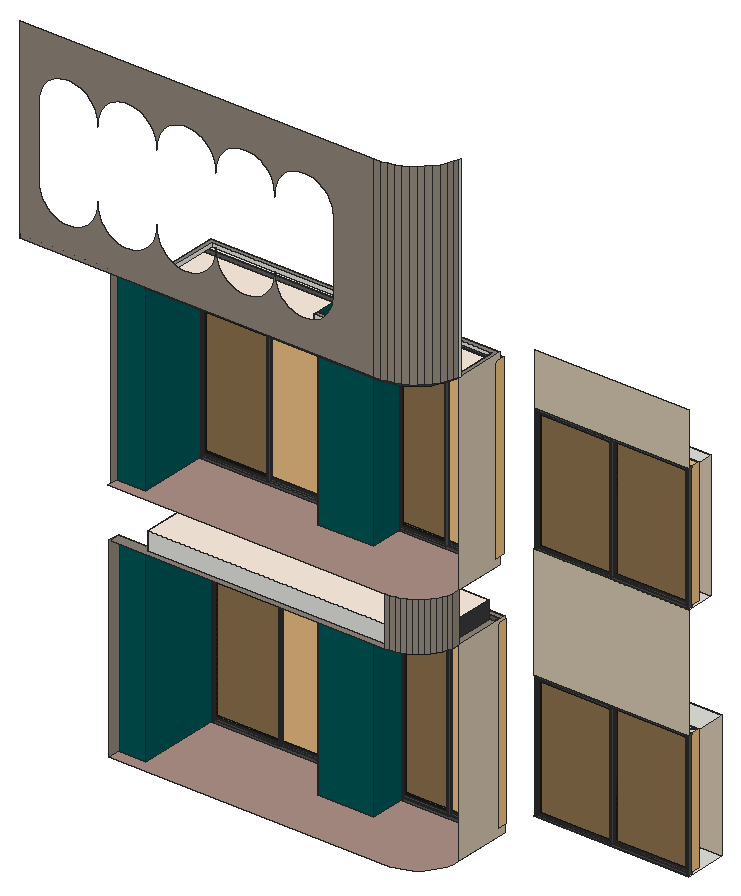
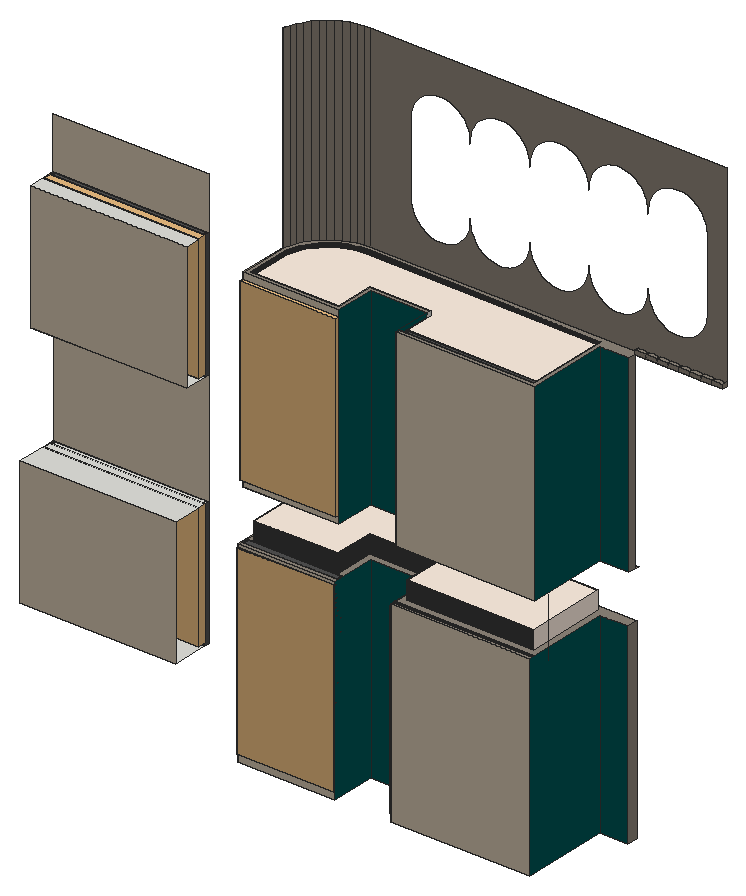
# SketchUp Ruby script. Lengths in inches.
U = 1.inch
M = Sketchup.active_model
def pt(a) = Geom::Point3d.new(a.map { |v| v * U })
def face(e, loops, mat)
  f = e.add_face(loops[0].map { |a| pt(a) })
  loops[1..].each { |l| e.add_face(l.map { |a| pt(a) }).erase! }
  f.material = f.back_material = mat if mat
  f
end
# faces: each face lists its corners as indices into pts; further lists are holes
def faces(e, pts, list, mat = nil) = list.each { |f| face(e, (f[0].is_a?(Array) ? f : [f]).map { |l| l.map { |i| pts[i] } }, mat) }
# xy, xz, yz: faces in a plane at the given z, y or x. An outline is a flat list of corners, or four numbers for a rectangle; further outlines are holes
def ring(l) = l.size == 4 ? [[l[0], l[1]], [l[2], l[1]], [l[2], l[3]], [l[0], l[3]]] : l.each_slice(2).to_a
def flat(e, list, mat, &to3) = list.each { |f| face(e, (f[0].is_a?(Array) ? f : [f]).map { |l| ring(l).map { |u, v| to3.(u, v) } }, mat) }
def xy(e, z, list, mat = nil) = flat(e, list, mat) { |x, y| [x, y, z] }
def xz(e, y, list, mat = nil) = flat(e, list, mat) { |x, z| [x, y, z] }
def yz(e, x, list, mat = nil) = flat(e, list, mat) { |y, z| [x, y, z] }
def lines(e, pts, list) = list.each { |a, b| e.add_line(pt(pts[a]), pt(pts[b])) }
# prism: a flat outline (further loops are holes) pulled along v
def prism(e, loops, v, mat = nil)
  f = face(e, loops, mat); d = Geom::Vector3d.new(v.map { |x| x * U })
  f.pushpull(f.normal.samedirection?(d) ? d.length : -d.length)
end
def box(e, o, s, mat = nil) = prism(e, [[o, [o[0] + s[0], o[1], o[2]], [o[0] + s[0], o[1] + s[1], o[2]], [o[0], o[1] + s[1], o[2]]]], [0, 0, s[2]], mat)
def at(x, y, z, deg = 0) = Geom::Transformation.translation(pt([x, y, z])) * Geom::Transformation.rotation(ORIGIN, Z_AXIS, deg.degrees)
def axes(o, x, y, z) = Geom::Transformation.new([*x, 0, *y, 0, *z, 0, *pt(o).to_a, 1])
def part(name) = M.definitions.add(name)
# library, detail: a bought-in or finely detailed component or shape, given as its bounding box
def library(name, o, s) = part(name).tap { |d| box(d.entities, o, s) }
def detail(e, o, s) = box(e.add_group.entities, o, s)
def put(e, d, t, mat = nil) = e.add_instance(d, t).tap { |i| i.material = mat if mat }
def group(e, t, mat = nil) = e.add_group.tap { |g| g.transformation = t; g.material = mat if mat }.entities
root = M.entities
M.materials.add("Brown Tiles 240cm").color = [174, 145, 135]
M.materials.add("Glass_Tinted_Gray").color = [0, 0, 0]
M.materials["Glass_Tinted_Gray"].alpha = 0.125
M.materials.add("Heather_Band").color = [142, 133, 122]
M.materials.add("Lily_Blonde").color = [209, 194, 173]
M.materials.add("[0135_DarkGray]").color = [81, 81, 81]
M.materials.add("[Color C02]").color = [255, 240, 226]
M.materials.add("[Color H08]").color = [0, 84, 84]
M.materials.add("[Color M07]").color = [58, 58, 58]
M.materials.add("[Mirror 02]").color = [229, 229, 229]
M.materials.add("[Terrazzo Light Blue]").color = [196, 214, 227]
c1 = library("Window curtains",[0,0,0],[14.46,147.43,135.83])
c2 = part("PENTEK_RP Fineline 50S_Sliding_DoorCase_E1")
box(c2.entities,[0,0,0],[1.51,3.66,99.27],"[0135_DarkGray]")
c3 = part("PENTEK_RP Fineline 50S_SlidingDooe_Case_E2")
box(c3.entities,[0,0,0],[96.25,3.66,1.51],"[0135_DarkGray]")
c4 = part("pentek_RP Fineline 50S_SlidingDoor_Case")
put(c4.entities,c2,at(97.76,0,0))
put(c4.entities,c3,at(1.51,0,0))
put(c4.entities,c2,at(0,0,0))
put(c4.entities,c3,at(1.51,0,97.76))
c5 = part("PENTEK_RP Fineline 50S_SlidingDoor_GlazingBead_2")
box(c5.entities,[0,0,0],[0.56,0.59,94.39],"[0135_DarkGray]")
c6 = part("PENTEK_RP Fineline 50S_SlidingDoor_Glass")
box(c6.entities,[0,0,0],[46.58,0.16,94.39],"Glass_Tinted_Gray")
c7 = part("PENTEK_RP Fineline 50S_SlidingDoor_GlazingBead")
box(c7.entities,[0,0,0],[45.47,0.59,0.56],"[0135_DarkGray]")
c8 = part("PENTEK_RP Fineline 50S_SlidingDoor_Leaf_E1")
xy(c8.entities,0,[[0,0,0.93,1.97],[0.93,1.57,1.49,1.97]],"[0135_DarkGray]")
xy(c8.entities,96.25,[[0,0,0.93,0,0.93,1.57,1.49,1.57,1.49,1.97,0,1.97]],"[0135_DarkGray]")
xz(c8.entities,0,[[0,0,0.93,96.25]],"[0135_DarkGray]")
xz(c8.entities,1.57,[[0.93,0,1.49,95.32],[0.93,95.32,1.49,96.25]],"[0135_DarkGray]")
xz(c8.entities,1.97,[[0,0,1.49,96.25]],"[0135_DarkGray]")
yz(c8.entities,0,[[0,0,1.97,96.25]],"[0135_DarkGray]")
yz(c8.entities,0.93,[[0,0,1.57,0.93],[0,0.93,1.57,95.32],[0,95.32,1.57,96.25]],"[0135_DarkGray]")
yz(c8.entities,1.49,[[1.57,0,1.97,95.32],[1.57,95.32,1.97,96.25]],"[0135_DarkGray]")
c9 = part("PENTEK_RP Fineline 50S_SlidingDoor_Leaf_E2")
xy(c9.entities,0,[[0,0,0,1.57,0.56,1.57,0.56,1.97,46.02,1.97,46.02,1.57,46.58,1.57,46.58,0]],"[0135_DarkGray]")
xy(c9.entities,0.93,[[0,0,46.58,1.57]],"[0135_DarkGray]")
xy(c9.entities,1.49,[[0.56,1.57,46.02,1.97]],"[0135_DarkGray]")
xz(c9.entities,0,[[0,0,46.58,0.93]],"[0135_DarkGray]")
xz(c9.entities,1.57,[[0,0,0.56,0.93],[46.02,0,46.58,0.93],[0.56,0.93,46.02,1.49]],"[0135_DarkGray]")
xz(c9.entities,1.97,[[0.56,0,46.02,1.49]],"[0135_DarkGray]")
yz(c9.entities,0,[[0,0,1.57,0.93]],"[0135_DarkGray]")
yz(c9.entities,0.56,[[1.57,0,1.97,0.93],[1.57,0.93,1.97,1.49]],"[0135_DarkGray]")
yz(c9.entities,46.02,[[1.57,0,1.97,0.93],[1.57,0.93,1.97,1.49]],"[0135_DarkGray]")
yz(c9.entities,46.58,[[0,0,1.57,0.93]],"[0135_DarkGray]")
c10 = part("PENTEK_RP Fineline S_SlidingDoor_Leaf1")
put(c10.entities,c5,at(0.93,0,0.93))
put(c10.entities,c5,at(46.96,0,0.93))
put(c10.entities,c6,at(1.49,1.42,0.93))
put(c10.entities,c7,at(1.49,0,0.93))
put(c10.entities,c6,at(1.49,0.59,0.93),"[Terrazzo Light Blue]")
put(c10.entities,c8,at(0,0,0))
put(c10.entities,c8,axes([48.44,0,0],[-1,0,0],[0,1,0],[0,0,1]))
put(c10.entities,c9,axes([0.93,0,96.25],[1,0,0],[0,1,0],[0,0,-1]))
put(c10.entities,c9,at(0.93,0,0))
put(c10.entities,c7,at(1.49,0,94.77))
c11 = part("PENTEK_RP Fineline 50S_SlidingDoor_Leaf2")
put(c11.entities,c6,at(1.49,1.42,0.93))
put(c11.entities,c7,at(1.49,0,94.77))
put(c11.entities,c5,at(46.96,0,0.93))
put(c11.entities,c6,at(1.49,0.59,0.93),"[Mirror 02]")
put(c11.entities,c5,at(0.93,0,0.93))
put(c11.entities,c8,at(0,0,0))
put(c11.entities,c8,axes([48.44,0,0],[-1,0,0],[0,1,0],[0,0,1]))
put(c11.entities,c7,at(1.49,0,0.93))
put(c11.entities,c9,axes([0.93,0,96.25],[1,0,0],[0,1,0],[0,0,-1]))
put(c11.entities,c9,at(0.93,0,0))
c12 = part("PENTEK - Slimmest Steel Sliding Door / Window\#1")
put(c12.entities,c4,at(0,-1.88,-0.09))
put(c12.entities,c10,at(1.51,-2.27,1.42))
put(c12.entities,c11,at(49.32,-0.3,1.42))
c13 = part("Group\#18")
put(c13.entities,c1,axes([0,8.14,5.43],[0,-0.42,0],[1.40442,0,0],[0,0,0.9702]))
put(c13.entities,c12,axes([0,2.27,0.13],[2.0736,0,0],[0,1,0],[0,0,1.4]))
c14 = library("White+Curtain+Sketchup",[0,-2.58,0],[59,4.99,76.02])
c15 = part("Group\#8")
put(c15.entities,c12,axes([0.12,3.91,0.18],[2.38,0,0],[0,1.72,0],[0,0,1.94621]))
put(c15.entities,c14,axes([0,13.43,3.17],[4.00656,0,0],[0,2.5,0],[0,0,2.5]))
xy(root,594.72,[[68.4,4.77,279.88,4.77,283.5,4.97,287.07,5.58,290.54,6.6,293.88,7.99,297.05,9.76,299.99,11.875,302.67,14.31,305.06,17.03,307.13,20,308.85,23.19,310.19,26.55,311.15,30.05,311.15,80.33,237.9,80.33,237.9,45.95,195.07,45.95,195.07,80.33,89.34,80.33,89.34,13.55,68.4,13.55]],"Brown Tiles 240cm")
xy(root,640.97,[[363.26,43.02,481.45,74.95]])
xy(root,737.58,[[363.26,43.02,481.45,74.95]])
xy(root,743.26,[[[68.4,4.77,68.4,13.55,89.34,13.55,89.34,80.33,195.07,80.33,195.07,45.95,237.9,45.95,237.9,80.33,311.15,80.33,311.15,30.05,310.19,26.55,308.85,23.19,307.13,20,305.06,17.03,302.67,14.31,299.99,11.875,297.05,9.76,293.88,7.99,290.54,6.6,287.07,5.58,283.5,4.97,279.88,4.77],[94.07,9.49,279.75,9.49,282.96,9.67,286,10.2,288.97,11.06,291.8125,12.25,294.5,13.76,297.01,15.56,299.3,17.63,301.33,19.95,303.09,22.48,304.56,25.2,305.71,28.0625,306.42,30.68,306.42,71.01,242.62,71.01,242.62,41.23,190.35,41.23,190.35,71.01,94.07,71.01]]],"Heather_Band")
xy(root,756.95,[[94.07,9.49,94.07,71.01,190.35,71.01,190.35,41.23,242.62,41.23,242.62,71.01,306.42,71.01,306.42,30.68,305.71,28.0625,304.56,25.2,303.09,22.48,301.33,19.95,299.3,17.63,297.01,15.56,294.5,13.76,291.8125,12.25,288.97,11.06,286,10.2,282.96,9.67,279.75,9.49]],"[Color C02]")
xy(root,780.59,[[67.06,4.77,279.88,4.77,283.5,4.97,287.07,5.58,290.54,6.6,293.88,7.99,297.05,9.76,299.99,11.875,302.67,14.31,305.06,17.03,307.13,20,308.85,23.19,310.19,26.55,311.15,30.05,311.15,75.73,237.9,75.73,237.9,45.95,195.07,45.95,195.07,75.73,89.34,75.73,89.34,13.55,67.06,13.55]],"Brown Tiles 240cm")
xy(root,824.16,[[363.26,43.02,481.45,64.39]])
xy(root,920.76,[[363.26,43.35,481.45,64.39]])
xy(root,923.32,[[92.75,8.18,92.75,72.32,195.07,72.32,195.07,42.54,241.31,42.54,241.31,72.32,307.74,72.32,307.74,37.97,306.75,34.07,305.24,30.09,303.28,26.3125,300.9,22.78,298.13,19.55,295.01,16.66,291.58,14.14,287.88,12.03,283.97,10.37,279.88,9.16,275.69,8.43,271.34,8.18]],"[Color C02]")
xy(root,926.45,[[0,4.77,0,8.08,67.06,8.08,67.06,13.55,89.34,13.55,89.34,75.73,195.07,75.73,195.07,72.32,92.75,72.32,92.75,8.18,271.34,8.18,275.69,8.43,279.88,9.16,283.97,10.37,287.88,12.03,291.58,14.14,295.01,16.66,298.13,19.55,300.9,22.78,303.28,26.3125,305.24,30.09,306.75,34.07,307.74,37.97,307.74,72.32,241.31,72.32,241.31,42.54,195.07,42.54,195.07,45.95,237.9,45.95,237.9,75.73,311.15,75.73,311.15,37.55,310.01,33.04,308.36,28.69,306.22,24.57,303.62,20.71,300.6,17.18,297.1875,14.02,293.4375,11.27,289.4,8.97,285.12,7.15,280.66,5.83,276.08,5.03,271.44,4.77]],"Heather_Band")
xy(root,929.63,[[4.19,5.14,3.83,5.16,3.47,5.2,3.11,5.27,2.76,5.375,2.42,5.51,2.1,5.66,1.78,5.85,1.49,6.06,1.21,6.29,0.95,6.54,0.71,6.82,0.49,7.11,0.3,7.42,0.14,7.74,0,8.08,8.38,8.08,8.24,7.74,8.08,7.42,7.89,7.11,7.67,6.82,7.4375,6.54,7.18,6.29,6.9,6.06,6.6,5.85,6.29,5.66,5.96,5.51,5.62,5.375,5.27,5.27,4.91,5.2,4.55,5.16],[12.57,5.14,12.21,5.16,11.85,5.2,11.49,5.27,11.14,5.375,10.81,5.51,10.48,5.66,10.16,5.85,9.87,6.06,9.59,6.29,9.33,6.54,9.09,6.82,8.875,7.11,8.68,7.42,8.52,7.74,8.38,8.08,16.76,8.08,16.625,7.74,16.46,7.42,16.27,7.11,16.06,6.82,15.82,6.54,15.56,6.29,15.28,6.06,14.98,5.85,14.67,5.66,14.34,5.51,14,5.375,13.65,5.27,13.3,5.2,12.9375,5.16],[20.95,5.14,20.59,5.16,20.23,5.2,19.875,5.27,19.53,5.375,19.1875,5.51,18.86,5.66,18.55,5.85,18.25,6.06,17.97,6.29,17.71,6.54,17.47,6.82,17.26,7.11,17.07,7.42,16.9,7.74,16.76,8.08,25.15,8.08,25.01,7.74,24.84,7.42,24.65,7.11,24.4375,6.82,24.2,6.54,23.94,6.29,23.66,6.06,23.36,5.85,23.05,5.66,22.72,5.51,22.38,5.375,22.03,5.27,21.68,5.2,21.32,5.16],[29.34,5.14,28.97,5.16,28.61,5.2,28.26,5.27,27.91,5.375,27.57,5.51,27.24,5.66,26.93,5.85,26.63,6.06,26.35,6.29,26.09,6.54,25.85,6.82,25.64,7.11,25.45,7.42,25.28,7.74,25.15,8.08,33.53,8.08,33.39,7.74,33.23,7.42,33.03,7.11,32.82,6.82,32.58,6.54,32.32,6.29,32.04,6.06,31.74,5.85,31.43,5.66,31.1,5.51,30.76,5.375,30.42,5.27,30.06,5.2,29.7,5.16],[37.72,5.14,37.36,5.16,37,5.2,36.64,5.27,36.29,5.375,35.95,5.51,35.625,5.66,35.3125,5.85,35.01,6.06,34.73,6.29,34.47,6.54,34.24,6.82,34.02,7.11,33.83,7.42,33.67,7.74,33.53,8.08,41.91,8.08,41.77,7.74,41.61,7.42,41.42,7.11,41.2,6.82,40.96,6.54,40.7,6.29,40.42,6.06,40.125,5.85,39.8125,5.66,39.49,5.51,39.15,5.375,38.8,5.27,38.44,5.2,38.08,5.16],
  [46.1,5.14,45.74,5.16,45.375,5.2,45.02,5.27,44.67,5.375,44.33,5.51,44.01,5.66,43.69,5.85,43.39,6.06,43.12,6.29,42.86,6.54,42.62,6.82,42.4,7.11,42.21,7.42,42.05,7.74,41.91,8.08,49.39,8.08,49.39,6.59,49.35,6.54,49.09,6.29,48.81,6.06,48.51,5.85,48.2,5.66,47.87,5.51,47.53,5.375,47.18,5.27,46.82,5.2,46.46,5.16],[54.48,5.14,54.12,5.16,53.76,5.2,53.4,5.27,53.05,5.375,52.72,5.51,52.39,5.66,52.07,5.85,51.78,6.06,51.5,6.29,51.24,6.54,51,6.82,50.78,7.11,50.59,7.42,50.43,7.74,50.29,8.08,58.67,8.08,58.54,7.74,58.37,7.42,58.18,7.11,57.97,6.82,57.73,6.54,57.47,6.29,57.1875,6.06,56.89,5.85,56.58,5.66,56.25,5.51,55.91,5.375,55.5625,5.27,55.21,5.2,54.85,5.16],[62.86,5.14,62.5,5.16,62.14,5.2,61.79,5.27,61.4375,5.375,61.1,5.51,60.77,5.66,60.46,5.85,60.16,6.06,59.88,6.29,59.62,6.54,59.38,6.82,59.17,7.11,58.98,7.42,58.8125,7.74,58.67,8.08,67.06,8.08,66.92,7.74,66.75,7.42,66.5625,7.11,66.35,6.82,66.11,6.54,65.85,6.29,65.57,6.06,65.27,5.85,64.96,5.66,64.63,5.51,64.29,5.375,63.94,5.27,63.59,5.2,63.23,5.16],[49.39,6.59,49.39,8.08,50.29,8.08,50.15,7.74,49.99,7.42,49.8,7.11,49.58,6.82]],"Heather_Band")
xz(root,4.77,[[[0,926.45,271.44,1076],[37.11,948.03,34.64,948.16,32.2,948.57,29.8125,949.24,27.52,950.17,25.34,951.34,23.3,952.74,21.42,954.36,19.73,956.17,18.26,958.16,17,960.29,15.99,962.55,15.23,964.91,14.74,967.34,14.55,969.34,14.51,969.8,14.55,972.28,14.55,969.34,14.51,969.8,14.55,972.28,14.55,1023.73,14.51,1026.21,14.55,1026.72,14.55,1023.73,14.51,1026.21,14.55,1026.72,14.73,1028.68,15.23,1031.11,15.98,1033.47,16.99,1035.73,18.24,1037.87,19.72,1039.86,21.41,1041.68,23.28,1043.3,25.33,1044.7,27.51,1045.875,29.81,1046.8,32.19,1047.47,34.64,1047.88,37.11,1048.02,39.59,1047.88,42.03,1047.47,44.42,1046.8,46.72,1045.875,48.9,1044.7,50.94,1043.3,52.82,1041.68,54.5,1039.86,55.98,1037.87,57.23,1035.73,58.24,1033.47,59,1031.11,59.5,1028.68,59.67,1026.72,59.72,1026.21,59.67,1023.73,59.67,1026.72,59.85,1028.68,60.35,1031.11,61.1,1033.47,62.11,1035.73,63.37,1037.87,64.84,1039.86,66.53,1041.68,68.41,1043.3,70.45,1044.7,72.63,1045.875,74.93,1046.8,77.32,1047.47,79.76,1047.88,82.24,1048.02,84.71,1047.88,87.15,1047.47,89.54,1046.8,91.84,1045.875,94.02,1044.7,96.0625,1043.3,97.9375,1041.68,99.625,1039.86,101.1,1037.87,102.36,1035.73,103.37,1033.47,104.125,1031.11,104.62,1028.68,104.8,1026.72,104.98,1028.68,105.47,1031.11,106.23,1033.47,107.24,1035.73,108.49,1037.87,109.97,1039.86,111.65,1041.68,113.53,1043.3,115.57,1044.7,117.75,1045.875,120.05,1046.8,122.4375,1047.47,124.88,1047.88,127.36,1048.02,129.83,1047.88,132.28,1047.47,134.66,1046.8,136.96,1045.875,139.14,1044.7,141.1875,1043.3,143.0625,1041.68,144.75,1039.86,146.23,1037.87,147.48,1035.73,148.49,1033.47,149.25,1031.11,149.74,1028.68,149.92,1026.72,150.1,1028.68,150.59,1031.11,151.35,1033.47,152.36,1035.73,153.61,1037.87,155.09,1039.86,156.78,1041.68,158.65,1043.3,160.69,1044.7,162.875,1045.875,165.17,1046.8,167.56,1047.47,170,1047.88,172.48,1048.02,174.95,1047.88,177.4,1047.47,179.78,1046.8,182.08,1045.875,184.27,1044.7,186.31,1043.3,188.18,1041.68,189.87,1039.86,191.35,1037.87,192.6,1035.73,193.61,1033.47,194.37,1031.11,194.86,1028.68,195.04,1026.72,195.22,1028.68,195.71,1031.11,196.47,1033.47,197.48,1035.73,198.73,1037.87,200.21,1039.86,201.9,1041.68,203.77,1043.3,205.8125,1044.7,208,1045.875,210.3,1046.8,212.68,1047.47,215.125,1047.88,217.6,1048.02,220.08,1047.88,222.52,1047.47,224.91,1046.8,227.2,1045.875,229.39,1044.7,231.43,1043.3,233.3,1041.68,234.99,1039.86,236.47,1037.87,237.72,1035.73,238.73,1033.47,239.49,1031.11,239.98,1028.68,240.16,1026.72,240.16,969.34,239.98,967.34,239.48,964.91,238.72,962.55,237.71,960.29,236.46,958.16,234.98,956.17,233.29,954.36,231.42,952.74,229.38,951.34,227.2,950.17,224.9,949.24,222.52,948.57,220.07,948.16,217.6,948.03,215.13,948.16,212.69,948.57,210.3,949.24,208,950.17,205.82,951.34,203.78,952.74,201.91,954.36,200.22,956.17,198.74,958.16,197.49,960.29,196.48,962.55,195.72,964.91,195.22,967.34,195.04,969.34,194.86,967.34,194.36,964.91,193.6,962.55,192.59,960.29,191.34,958.16,189.86,956.17,188.17,954.36,186.3,952.74,184.26,951.34,182.08,950.17,179.78,949.24,177.39,948.57,174.95,948.16,172.48,948.03,170.01,948.16,167.5625,948.57,165.18,949.24,162.88,950.17,160.7,951.34,158.66,952.74,156.79,954.36,155.1,956.17,153.62,958.16,152.37,960.29,151.36,962.55,150.6,964.91,150.1,967.34,149.92,969.34,149.73,967.34,149.24,964.91,148.48,962.55,147.47,960.29,146.21,958.16,144.74,956.17,143.05,954.36,141.18,952.74,139.13,951.34,136.95,950.17,134.66,949.24,132.27,948.57,129.83,948.16,127.36,948.03,124.88,948.16,122.44,948.57,120.06,949.24,117.76,950.17,115.58,951.34,113.54,952.74,111.66,954.36,109.98,956.17,108.5,958.16,107.25,960.29,106.24,962.55,105.48,964.91,104.98,967.34,104.8,969.34,104.61,967.34,104.12,964.91,103.36,962.55,102.35,960.29,101.09,958.16,99.61,956.17,97.93,954.36,96.05,952.74,94.01,951.34,91.83,950.17,89.53,949.24,87.15,948.57,84.71,948.16,82.24,948.03,79.76,948.16,77.32,948.57,74.9375,949.24,72.64,950.17,70.46,951.34,68.42,952.74,66.54,954.36,64.86,956.17,63.38,958.16,62.125,960.29,61.11,962.55,60.36,964.91,59.86,967.34,59.67,969.34,59.67,972.28,59.72,969.8,59.67,969.34,59.49,967.34,58.99,964.91,58.23,962.55,57.22,960.29,55.97,958.16,54.49,956.17,52.81,954.36,50.93,952.74,48.89,951.34,46.71,950.17,44.41,949.24,42.03,948.57,39.59,948.16],[104.8,1023.73,104.8,1026.72,104.84,1026.21],[149.92,1023.73,149.92,1026.72,149.96,1026.21],[195.04,1023.73,195.04,1026.72,195.09,1026.21],[149.92,969.34,149.92,972.28,149.96,969.8],[104.8,969.34,104.8,972.28,104.84,969.8],[195.04,969.34,195.04,972.28,195.08,969.8]]],"Heather_Band")
xz(root,8.08,[[0,926.45,8.38,929.63],[8.38,926.45,16.76,929.63],[16.76,926.45,25.15,929.63],[25.15,926.45,33.53,929.63],[33.53,926.45,41.91,929.63],
  [41.91,926.45,50.29,929.63],[50.29,926.45,58.67,929.63],[58.67,926.45,67.06,929.63]],"Heather_Band")
xz(root,8.18,[[92.75,923.32,271.34,926.45]],"[Color M07]")
xz(root,9.49,[[94.07,743.26,279.75,756.95]])
xz(root,13.55,[[68.4,594.72,89.34,743.26],[67.06,780.59,89.34,926.45]],"[Color H08]")
xz(root,41.23,[[190.35,743.26,242.62,756.95]],"[Color M07]")
xz(root,42.54,[[195.07,923.32,241.31,926.45]])
xz(root,43.02,[[363.26,737.58,481.45,824.16]],"Lily_Blonde")
xz(root,43.35,[[363.26,920.76,481.45,960.77]],"Lily_Blonde")
xz(root,45.95,[[195.07,594.72,237.9,743.26],[195.07,780.59,237.9,926.45]],"[Color H08]")
xz(root,64.39,[[363.26,824.16,481.45,920.76]],"Lily_Blonde")
xz(root,71.01,[[94.07,743.26,190.35,756.95],[242.62,743.26,306.42,756.95]],"[Color M07]")
xz(root,72.32,[[92.75,923.32,195.07,926.45],[241.31,923.32,307.74,926.45]])
xz(root,74.95,[[363.26,640.97,481.45,737.58]],"Lily_Blonde")
xz(root,75.73,[[89.34,780.59,195.07,926.45],[237.9,780.59,311.15,926.45]],"Lily_Blonde")
xz(root,80.33,[[89.34,594.72,195.07,743.26],[237.9,594.72,311.15,743.26]],"Lily_Blonde")
yz(root,0,[[4.77,926.45,8.08,929.63]],"Heather_Band")
yz(root,67.06,[[8.08,780.59,13.55,926.45]],"Heather_Band")
yz(root,68.4,[[4.77,594.72,13.55,743.26]],"Heather_Band")
yz(root,89.34,[[13.55,594.72,80.33,743.26],[13.55,780.59,75.73,926.45]],"[Color H08]")
yz(root,92.75,[[8.18,923.32,13.55,926.45],[13.55,923.32,72.32,926.45]])
yz(root,94.07,[[9.49,743.26,71.01,756.95]],"[Color C02]")
yz(root,190.35,[[41.23,743.26,71.01,756.95]],"[Color M07]")
yz(root,195.07,[[42.54,923.32,45.95,926.45]])
yz(root,195.07,[[45.95,594.72,80.33,743.26],[45.95,780.59,45.95,923.32,72.32,923.32,72.32,926.45,75.73,926.45,75.73,780.59],[45.95,923.32,72.32,926.45]],"[Color H08]")
yz(root,237.9,[[45.95,594.72,80.33,743.26],[45.95,780.59,75.73,926.45]],"[Color H08]")
yz(root,241.31,[[42.54,923.32,72.32,926.45]])
yz(root,242.62,[[41.23,743.26,71.01,756.95]],"[Color M07]")
yz(root,306.42,[[30.68,743.26,35.95,756.95]])
yz(root,306.42,[[35.95,743.26,71.01,756.95]],"[Color M07]")
yz(root,307.74,[[37.97,923.32,72.32,926.45]],"[Color M07]")
yz(root,311.15,[[35.95,926.45,37.55,1076]])
yz(root,311.15,[[30.05,743.26,35.95,780.59]],"Heather_Band")
yz(root,311.15,[[35.95,594.72,80.33,743.26],[35.95,780.59,75.73,926.45]],"Lily_Blonde")
p = [[283.5,4.97,780.59],[279.88,4.77,780.59],[279.88,4.77,743.26],[283.5,4.97,743.26],[287.07,5.58,780.59],[287.07,5.58,743.26],
  [290.54,6.6,780.59],[290.54,6.6,743.26],[293.88,7.99,780.59],[293.88,7.99,743.26],[297.05,9.76,780.59],[297.05,9.76,743.26],
  [282.96,9.67,743.26],[279.75,9.49,743.26],[279.75,9.49,756.95],[282.96,9.67,756.95],[286,10.2,743.26],[286,10.2,756.95],
  [299.99,11.875,780.59],[299.99,11.875,743.26],[288.97,11.06,743.26],[288.97,11.06,756.95],[291.8125,12.25,743.26],[291.8125,12.25,756.95],
  [302.67,14.31,780.59],[302.67,14.31,743.26],[294.5,13.76,743.26],[294.5,13.76,756.95],[297.01,15.56,743.26],[297.01,15.56,756.95],
  [305.06,17.03,780.59],[305.06,17.03,743.26],[299.3,17.63,743.26],[299.3,17.63,756.95],[307.13,20,780.59],[307.13,20,743.26],
  [301.33,19.95,743.26],[301.33,19.95,756.95],[303.09,22.48,743.26],[303.09,22.48,756.95],[308.85,23.19,780.59],[308.85,23.19,743.26],
  [304.56,25.2,743.26],[304.56,25.2,756.95],[310.19,26.55,780.59],[310.19,26.55,743.26],[305.71,28.0625,743.26],[305.71,28.0625,756.95],
  [311.15,30.05,780.59],[311.15,30.05,743.26],[306.42,30.68,743.26],[306.42,30.68,756.95],[275.69,8.43,926.45],[271.34,8.18,926.45],
  [271.34,8.18,923.32],[275.69,8.43,923.32],[279.88,9.16,926.45],[279.88,9.16,923.32],[283.97,10.37,926.45],[283.97,10.37,923.32],
  [287.88,12.03,926.45],[287.88,12.03,923.32],[291.58,14.14,926.45],[291.58,14.14,923.32],[295.01,16.66,926.45],[295.01,16.66,923.32],
  [298.13,19.55,926.45],[298.13,19.55,923.32],[300.9,22.78,926.45],[300.9,22.78,923.32],[303.28,26.3125,926.45],[303.28,26.3125,923.32],
  [305.24,30.09,926.45],[305.24,30.09,923.32],[306.75,34.07,926.45],[306.75,34.07,923.32],[307.74,37.97,926.45],[307.74,37.97,923.32],
  [276.08,5.03,1076],[271.44,4.77,1076],[271.44,4.77,926.45],[276.08,5.03,926.45],[280.66,5.83,1076],[280.66,5.83,926.45],
  [285.12,7.15,1076],[285.12,7.15,926.45],[289.4,8.97,1076],[289.4,8.97,926.45],[293.4375,11.27,1076],[293.4375,11.27,926.45],
  [297.1875,14.02,1076],[297.1875,14.02,926.45],[300.6,17.18,1076],[300.6,17.18,926.45],[303.62,20.71,1076],[303.62,20.71,926.45],
  [306.22,24.57,1076],[306.22,24.57,926.45],[308.36,28.69,1076],[308.36,28.69,926.45],[310.01,33.04,1076],[310.01,33.04,926.45],
  [311.15,37.55,1076],[311.15,37.55,926.45],[79,75.73,743.26],[79,75.73,788.55],[50.29,8.08,929.63],[50.29,4.77,929.63],
  [58.67,8.08,929.63],[58.67,4.77,929.63],[67.06,8.08,929.63],[67.06,4.77,929.63],[41.91,8.08,929.63],[41.91,4.77,929.63],
  [8.38,8.08,929.63],[8.38,4.77,929.63],[16.76,8.08,929.63],[16.76,4.77,929.63],[25.15,8.08,929.63],[25.15,4.77,929.63],
  [33.53,8.08,929.63],[33.53,4.77,929.63],[49.39,6.59,929.63],[49.39,4.77,929.63]]
faces(root,p,[[0,1,2,3],[4,0,3,5],[6,4,5,7],[8,6,7,9],[10,8,9,11],[18,10,11,19],[24,18,19,25],[30,24,25,31],
  [34,30,31,35],[40,34,35,41],[44,40,41,45],[48,44,45,49],[78,79,80,81],[82,78,81,83],[84,82,83,85],[86,84,85,87],
  [88,86,87,89],[90,88,89,91],[92,90,91,93],[94,92,93,95],[96,94,95,97],[98,96,97,99],[100,98,99,101],[102,100,101,103]],"Heather_Band")
faces(root,p,[[12,13,14,15],[16,12,15,17],[20,16,17,21],[22,20,21,23],[26,22,23,27],[28,26,27,29],[32,28,29,33],[36,32,33,37],
  [38,36,37,39],[42,38,39,43],[46,42,43,47],[50,46,47,51]])
faces(root,p,[[52,53,54,55],[56,52,55,57],[58,56,57,59],[60,58,59,61],[62,60,61,63],[64,62,63,65],[66,64,65,67],[68,66,67,69],
  [70,68,69,71],[72,70,71,73],[74,72,73,75],[76,74,75,77]],"[Color M07]")
lines(root,p,[[104,105],[106,107],[108,109],[110,111],[112,113],[114,115],[116,117],[118,119],[120,121],[122,123]])
put(root,c13,axes([237.9,71.87,594.72],[0.35379,0,0],[0,1.15221,0],[0,0,1.06883]))
put(root,c13,axes([89.54,76.04,594.72],[0.51267,0,0],[0,0.5,0],[0,0,1.06883]))
put(root,c15,axes([363.26,43.02,640.97],[0.5,0,0],[0,0.5,0],[0,0,0.5]))
put(root,c13,axes([89.34,64.99,780.59],[0.51064,0,0],[0,1.15221,0],[0,0,1.02701]))
put(root,c13,axes([237.9,69.34,780.96],[0.35379,0,0],[0,1.15221,0],[0,0,1.02701]))
put(root,c15,axes([363.26,43.02,824.16],[0.5,0,0],[0,0.5,0],[0,0,0.5]))
